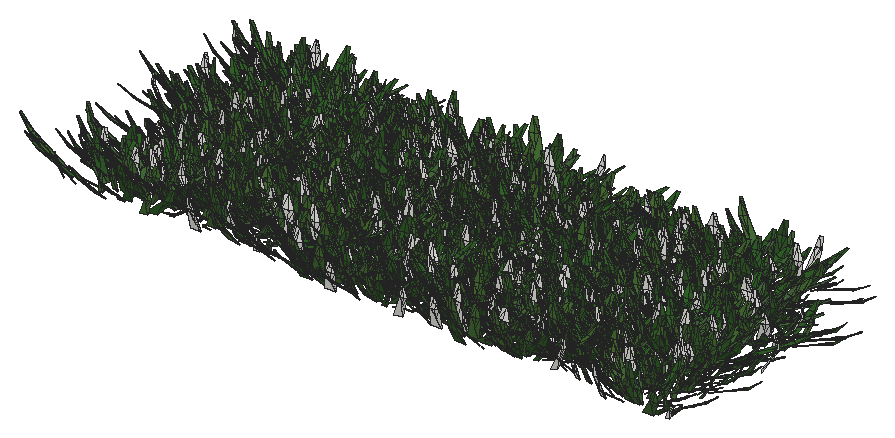
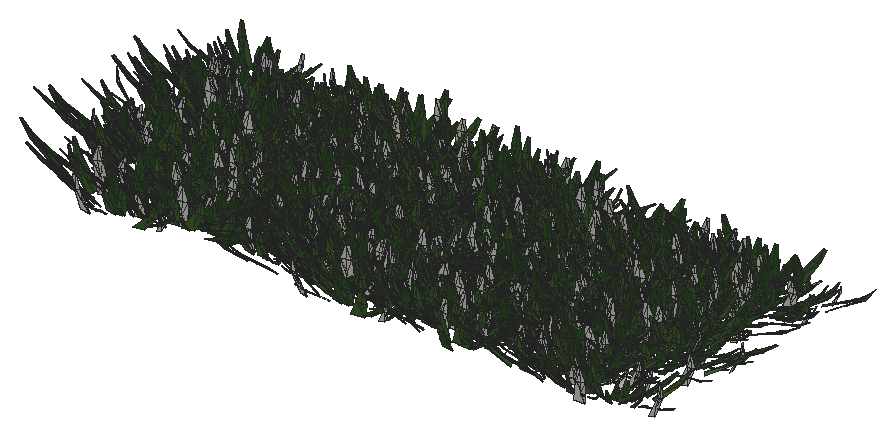
# SketchUp Ruby script. Lengths in inches.
U = 1.inch
M = Sketchup.active_model
def pt(a) = Geom::Point3d.new(a.map { |v| v * U })
def face(e, loops, mat)
  f = e.add_face(loops[0].map { |a| pt(a) })
  loops[1..].each { |l| e.add_face(l.map { |a| pt(a) }).erase! }
  f.material = f.back_material = mat if mat
  f
end
# faces: each face lists its corners as indices into pts; further lists are holes
def faces(e, pts, list, mat = nil) = list.each { |f| face(e, (f[0].is_a?(Array) ? f : [f]).map { |l| l.map { |i| pts[i] } }, mat) }
# xy, xz, yz: faces in a plane at the given z, y or x. An outline is a flat list of corners, or four numbers for a rectangle; further outlines are holes
def ring(l) = l.size == 4 ? [[l[0], l[1]], [l[2], l[1]], [l[2], l[3]], [l[0], l[3]]] : l.each_slice(2).to_a
def flat(e, list, mat, &to3) = list.each { |f| face(e, (f[0].is_a?(Array) ? f : [f]).map { |l| ring(l).map { |u, v| to3.(u, v) } }, mat) }
def xy(e, z, list, mat = nil) = flat(e, list, mat) { |x, y| [x, y, z] }
def xz(e, y, list, mat = nil) = flat(e, list, mat) { |x, z| [x, y, z] }
def yz(e, x, list, mat = nil) = flat(e, list, mat) { |y, z| [x, y, z] }
def lines(e, pts, list) = list.each { |a, b| e.add_line(pt(pts[a]), pt(pts[b])) }
# prism: a flat outline (further loops are holes) pulled along v
def prism(e, loops, v, mat = nil)
  f = face(e, loops, mat); d = Geom::Vector3d.new(v.map { |x| x * U })
  f.pushpull(f.normal.samedirection?(d) ? d.length : -d.length)
end
def box(e, o, s, mat = nil) = prism(e, [[o, [o[0] + s[0], o[1], o[2]], [o[0] + s[0], o[1] + s[1], o[2]], [o[0], o[1] + s[1], o[2]]]], [0, 0, s[2]], mat)
def at(x, y, z, deg = 0) = Geom::Transformation.translation(pt([x, y, z])) * Geom::Transformation.rotation(ORIGIN, Z_AXIS, deg.degrees)
def axes(o, x, y, z) = Geom::Transformation.new([*x, 0, *y, 0, *z, 0, *pt(o).to_a, 1])
def part(name) = M.definitions.add(name)
# library, detail: a bought-in or finely detailed component or shape, given as its bounding box
def library(name, o, s) = part(name).tap { |d| box(d.entities, o, s) }
def detail(e, o, s) = box(e.add_group.entities, o, s)
def put(e, d, t, mat = nil) = e.add_instance(d, t).tap { |i| i.material = mat if mat }
def group(e, t, mat = nil) = e.add_group.tap { |g| g.transformation = t; g.material = mat if mat }.entities
root = M.entities
M.materials.add("Material82").color = [68, 110, 58]
M.materials.add("Material83").color = [48, 90, 38]
M.materials.add("Material84").color = [68, 110, 48]
M.materials.add("Material85").color = [48, 90, 48]
M.materials.add("Material86").color = [58, 110, 58]
M.materials.add("Material87").color = [58, 90, 38]
M.materials.add("Material88").color = [68, 100, 58]
M.materials.add("Material89").color = [48, 100, 38]
c1 = part("grass00")
p = [[-0.6875,0.15,0],[-0.56,0.08,5.52],[-0.04,0.03,2.76],[0.48,-0.02,0],[0.35,-0.02,5.52],[-0.1,-0.14,5.52],
  [-0.12,0.65,8.37],[-0.42,0.65,8.37]]
faces(c1.entities,p,[[0,1,2,3],[3,2,4],[1,5,2],[5,4,2],[1,6,5],[4,5,6],[7,6,1]])
c2 = part("Group16\#1")
put(c2.entities,c1,axes([1.44,-0.61,-0.01],[0.05352,0.12609,0],[-0.10704,0.04543,0.07239],[0.06664,-0.02828,0.11628]),"Material85")
put(c2.entities,c1,axes([0.76,-0.15,-0.01],[0.04676,0.24062,0],[-0.23162,0.04501,0.06642],[0.0652,-0.01267,0.23595]),"Material82")
put(c2.entities,c1,axes([0.79,0.01,-0.01],[-0.00606,0.34651,0],[-0.34381,-0.00602,0.0432],[0.04319,0.00076,0.34386]))
put(c2.entities,c1,axes([1,0.23,-0.01],[-0.07192,0.31144,0],[-0.28722,-0.06632,0.1236],[0.12043,0.02781,0.29478]),"Material84")
put(c2.entities,c1,axes([1.66,0.77,-0.01],[-0.13828,0.29651,0],[-0.21551,-0.1005,0.22471],[0.20365,0.09498,0.23779]),"Material89")
put(c2.entities,c1,axes([0.6875,0.52,-0.01],[-0.18126,0.24051,0],[-0.22746,-0.17142,0.09788],[0.07817,0.05891,0.28481]),"Material84")
put(c2.entities,c1,axes([0.68,0.78,-0.01],[-0.215,0.18688,0],[-0.12385,-0.14248,0.21334],[0.13995,0.16101,0.18878]),"Material82")
put(c2.entities,c1,axes([0.56,1,-0.01],[-0.13756,0.07624,0],[-0.06159,-0.11112,0.0927],[0.04494,0.08108,0.12705]),"Material84")
put(c2.entities,c1,axes([0.2,0.64,-0.01],[-0.23729,0.07254,0],[-0.05711,-0.18681,0.153],[0.04473,0.14632,0.19535]),"Material89")
put(c2.entities,c1,axes([0.0625,0.72,-0.01],[-0.28874,0.02525,0],[-0.02179,-0.24916,0.14647],[0.01276,0.14591,0.25012]),"Material82")
put(c2.entities,c1,axes([-0.08,0.62,-0.01],[-0.34089,-0.04187,0],[0.03255,-0.26504,0.216],[-0.02633,0.21439,0.26703]),"Material89")
put(c2.entities,c1,axes([-0.34,0.98,-0.01],[-0.14314,-0.0493,0],[0.04397,-0.12769,0.06843],[-0.02228,0.0647,0.13505]),"Material89")
put(c2.entities,c1,axes([-0.87,1.45,-0.01],[-0.23488,-0.14114,0],[0.13761,-0.22901,0.06087],[-0.03135,0.05217,0.26717]))
put(c2.entities,c1,axes([-0.72,0.77,-0.01],[-0.14208,-0.13251,0],[0.07209,-0.0773,0.16301],[-0.11118,0.11922,0.1057]),"Material89")
put(c2.entities,c1,axes([-0.62,0.43,-0.01],[-0.14845,-0.21203,0],[0.18654,-0.13061,0.12304],[-0.10079,0.07057,0.22772]),"Material82")
put(c2.entities,c1,axes([-0.68,0.29,-0.01],[-0.13639,-0.32136,0],[0.31723,-0.13464,0.05579],[-0.05136,0.0218,0.34462]),"Material83")
put(c2.entities,c1,axes([-0.64,0.125,-0.01],[-0.0458,-0.23569,0],[0.22124,-0.043,0.08276],[-0.08124,0.01579,0.22538]),"Material86")
put(c2.entities,c1,axes([-1.6,-0.03,-0.01],[0.00576,-0.32897,0],[0.27526,0.00482,0.18018],[-0.18015,-0.00315,0.2753]),"Material84")
put(c2.entities,c1,axes([-1.36,-0.31,-0.01],[0.05718,-0.24765,0],[0.18172,0.04196,0.17267],[-0.16825,-0.03885,0.1865]),"Material89")
put(c2.entities,c1,axes([-1.54,-0.72,-0.01],[0.06537,-0.14017,0],[0.13555,0.06321,0.03939],[-0.0357,-0.01665,0.14956]))
put(c2.entities,c1,axes([-1.19,-0.9,-0.01],[0.09597,-0.12735,0],[0.11214,0.08451,0.07557],[-0.06035,-0.04548,0.14042]),"Material88")
put(c2.entities,c1,axes([-0.47,-0.54,-0.01],[0.11588,-0.10072,0],[0.0618,0.0711,0.12124],[-0.07953,-0.0915,0.0942]))
put(c2.entities,c1,axes([-0.47,-0.84,-0.01],[0.11927,-0.0661,0],[0.06603,0.11913,0.00646],[-0.00313,-0.00565,0.13621]),"Material84")
put(c2.entities,c1,axes([-0.38,-1.24,-0.01],[0.28037,-0.08571,0],[0.0618,0.20215,0.20315],[-0.05939,-0.19428,0.21139]),"Material88")
put(c2.entities,c1,axes([-0.06,-0.66,-0.01],[0.22719,-0.01987,0],[0.01247,0.14255,0.17758],[-0.01547,-0.17691,0.1431]),"Material87")
put(c2.entities,c1,axes([0.11,-0.89,-0.01],[0.14882,0.01828,0],[-0.01058,0.08611,0.12229],[0.01491,-0.12138,0.08676]),"Material85")
put(c2.entities,c1,axes([0.25,-0.72,-0.01],[0.20481,0.07053,0],[-0.06206,0.18022,0.10291],[0.03351,-0.0973,0.1906]),"Material85")
put(c2.entities,c1,axes([0.85,-1.42,-0.01],[0.16481,0.09904,0],[-0.09472,0.15762,0.05616],[0.02893,-0.04814,0.18389]),"Material84")
put(c2.entities,c1,axes([1.01,-1.09,-0.01],[0.21858,0.20385,0],[-0.17495,0.1876,0.15339],[0.10462,-0.11218,0.25652]),"Material89")
put(c2.entities,c1,axes([1.01,-0.71,-0.01],[0.08733,0.12473,0],[-0.06445,0.04512,0.13037],[0.1068,-0.07477,0.07867]),"Material85")
c3 = part("Group15\#1")
put(c3.entities,c2,at(0,0,0))
c4 = part("3darcstudiotree_grass00\#1")
put(c4.entities,c3,at(0,0,0))
put(root,c4,axes([773.21,342.86,-34.17],[3.14963,-1.20842,0],[2.29792,0.93151,-0.01443],[0.07601,0.03081,1.86565]))
put(root,c4,axes([774.36,356.8,-34.17],[-4.00454,-0.52801,0],[1.05814,-1.24816,-0.00172],[0.00311,-0.00367,1.42531]))
put(root,c4,axes([774.46,343.67,-34.17],[-1.0046,-1.54951,0],[3.94346,-0.39764,-0.04783],[0.24428,-0.02463,1.6084]))
put(root,c4,axes([772.96,366.74,-34.17],[2.75664,0.78459,0],[-2.60411,1.42301,-0.01696],[-0.0547,0.02989,1.8379]))
put(root,c4,axes([773.18,355.92,-34.17],[1.57656,1.15501,0],[-3.7913,0.80487,-0.00648],[-0.02974,0.00631,1.68262]))
put(root,c4,axes([775.48,345.66,-34.17],[-0.37683,-1.42813,0],[4.6236,-0.18974,-0.00351],[0.01488,-0.00061,1.48465]))
put(root,c4,axes([773.68,340.73,-34.17],[4.54007,0.12562,0],[-0.30482,1.71344,-0.05051],[-0.02069,0.11631,1.91076]))
put(root,c4,axes([775.09,350.05,-34.17],[1.62707,-1.18617,0],[3.8873,0.82932,-0.03985],[0.15889,0.0339,1.5017]))
put(root,c4,axes([774.64,359.32,-34.17],[4.17569,0.70475,0],[-1.86329,1.71705,-0.06274],[-0.13365,0.12316,1.92197]))
put(root,c4,axes([777.05,351.61,-34.17],[-3.80347,-0.79702,0],[1.88494,-1.39901,-0.03648],[0.10192,-0.07565,1.79293]))
put(root,c4,axes([776.98,349.31,-34.17],[-2.17021,-1.46243,0],[2.84473,-0.65657,-0.0221],[0.14072,-0.03248,1.82262]))
put(root,c4,axes([778.55,353.74,-34.17],[-2.18591,-1.17845,0],[3.11783,-0.89946,-0.02018],[0.10185,-0.02938,1.81061]))
put(root,c4,axes([777.24,367.79,-34.17],[4.09864,-0.14348,0],[0.37168,1.65134,-0.01913],[0.00999,0.04439,1.86132]))
put(root,c4,axes([777.85,355.56,-34.17],[-1.78032,1.61918,0],[-3.86174,-0.66038,-0.00354],[-0.01693,-0.0029,1.64409]))
put(root,c4,axes([778.8,342.72,-34.17],[3.03313,0.50579,0],[-1.37798,1.28522,-0.04149],[-0.11611,0.10829,1.90578]))
put(root,c4,axes([778.73,343.85,-34.17],[4.0409,0.57443,0],[-1.45336,1.59011,-0.05978],[-0.09434,0.10321,1.49495]))
put(root,c4,axes([778.6,364.67,-34.17],[3.09052,1.16305,0],[-2.75216,1.13741,-0.00767],[-0.03246,0.01341,1.8325]))
put(root,c4,axes([779.77,346.72,-34.17],[1.55138,-1.30688,0],[2.99369,0.55272,-0.04141],[0.29892,0.05519,1.97468]))
put(root,c4,axes([779.62,360.0625,-34.17],[4.14328,-0.46419,0],[1.00154,1.39037,-0.02465],[0.03463,0.04808,1.41248]))
put(root,c4,axes([780.14,358.2,-34.17],[-0.77153,1.33479,0],[-3.28421,-0.29525,-0.03421],[-0.24787,-0.02228,1.87625]))
put(root,c4,axes([780.48,361.74,-34.17],[-1.91367,1.54924,0],[-4.25661,-0.81775,-0.00711],[-0.02422,-0.00465,1.34501]))
put(root,c4,axes([781.09,366.36,-34.17],[3.43874,0.27286,0],[-0.6732,1.31953,-0.0192],[-0.02432,0.04768,1.64321]))
put(root,c4,axes([782.6,343.8125,-34.17],[-4.1133,-0.05921,0],[0.15009,-1.6218,-0.04384],[0.00865,-0.09349,1.66887]))
put(root,c4,axes([783.42,341.69,-34.17],[-3.5543,0.89209,0],[-1.79933,-1.11498,-0.04609],[-0.16829,-0.10428,1.7083]))
put(root,c4,axes([784.125,346.45,-34.17],[-2.34222,-1.01748,0],[3.28821,-1.17726,-0.05879],[0.21723,-0.07777,1.66118]))
put(root,c4,axes([783.17,363.76,-34.17],[3.65348,-0.50094,0],[1.24961,1.41744,-0.02118],[0.04225,0.04793,1.73224]))
put(root,c4,axes([784.34,359.43,-34.17],[-0.28709,-1.61704,0],[4.14071,-0.11434,-0.04142],[0.22933,-0.00633,1.72685]))
put(root,c4,axes([783.02,366.19,-34.17],[1.27855,1.29921,0],[-4.02019,0.61532,-0.04732],[-0.19364,0.02964,1.41896]))
put(root,c4,axes([783.54,350.0625,-34.17],[-1.96915,1.54328,0],[-4.06414,-0.80652,-0.00338],[-0.01619,-0.00321,1.82725]))
put(root,c4,axes([785.07,349.04,-34.17],[-3.56597,0.54096,0],[-1.21057,-1.24113,-0.01112],[-0.02689,-0.02757,1.70172]))
put(root,c4,axes([783.88,361.6,-34.17],[3.55843,0.77732,0],[-2.07504,1.47739,-0.02111],[-0.0608,0.04329,1.90804]))
put(root,c4,axes([784.41,357.15,-34.17],[4.24476,0.21314,0],[-0.43337,1.34235,-0.04636],[-0.04216,0.1306,1.85211]))
put(root,c4,axes([786.4,354.75,-34.17],[-3.8899,-0.78174,0],[2.11548,-1.63718,-0.02171],[0.04442,-0.03438,1.57387]))
put(root,c4,axes([786.41,353.11,-34.17],[3.28347,0.12106,0],[-0.38901,1.64106,-0.04931],[-0.02254,0.09507,1.538]))
put(root,c4,axes([789.21,354.72,-34.17],[-3.55041,0.9087,0],[-2.02381,-1.22981,-0.02727],[-0.0752,-0.0457,1.41127]))
put(root,c4,axes([788.76,359.69,-34.17],[1.12356,1.5327,0],[-3.46853,0.39546,-0.04889],[-0.25471,0.02904,1.46761]))
put(root,c4,axes([790.3125,344.57,-34.17],[1.64327,-1.14246,0],[4.09949,0.91708,-0.03953],[0.17253,0.0386,1.77239]))
put(root,c4,axes([789.09,342.6,-34.17],[0.41174,1.83159,0],[-3.96576,0.13865,-0.0152],[-0.08151,0.00285,1.60635]))
put(root,c4,axes([791.24,348.04,-34.17],[0.23576,-1.73441,0],[4.70751,0.09952,-0.00697],[0.03732,0.00079,1.89407]))
put(root,c4,axes([791.03,352.72,-34.17],[-3.49986,-0.57002,0],[1.44663,-1.38143,-0.04671],[0.11633,-0.11108,1.85324]))
put(root,c4,axes([790.11,346.12,-34.17],[0.9145,1.75116,0],[-3.69114,0.2998,-0.03105],[-0.20233,0.01643,1.87912]))
put(root,c4,axes([790.38,350.85,-34.17],[1.28043,1.73979,0],[-3.30316,0.37809,-0.03743],[-0.19576,0.02241,1.40382]))
put(root,c4,axes([790.87,361.54,-34.17],[2.41483,0.92576,0],[-3.06998,1.24547,-0.04673],[-0.14351,0.05822,1.45453]))
put(root,c4,axes([791.32,363.54,-34.17],[4.28624,-0.48224,0],[1.29741,1.79351,-0.04256],[0.05122,0.07081,1.55488]))
put(root,c4,axes([791.65,365.39,-34.17],[0.63995,1.63517,0],[-3.50377,0.21327,-0.04631],[-0.28502,0.01735,1.65491]))
put(root,c4,axes([792.12,357.61,-34.17],[4.08655,-0.74198,0],[1.4526,1.2443,-0.00355],[0.00912,0.00781,1.60125]))
put(root,c4,axes([792.1,367.56,-34.17],[1.05791,1.29898,0],[-3.4169,0.4328,-0.04361],[-0.24845,0.03147,1.60948]))
put(root,c4,axes([793.73,355.39,-34.17],[-0.24051,-1.38856,0],[3.98568,-0.10737,-0.04502],[0.19517,-0.00526,1.30109]))
put(root,c4,axes([794.77,344.86,-34.17],[1.00632,-1.60929,0],[3.83281,0.37276,-0.00763],[0.0458,0.00445,1.82848]))
put(root,c4,axes([795.37,350.2,-34.17],[-2.49579,-0.85332,0],[2.16334,-0.98408,-0.00893],[0.04692,-0.02134,1.98619]))
put(root,c4,axes([795.32,364.02,-34.17],[2.15184,-1.02148,0],[3.44742,1.1295,-0.00974],[0.03611,0.01183,1.619]))
put(root,c4,axes([795.6875,352.47,-34.17],[-3.56783,-0.13568,0],[0.42403,-1.73414,-0.0118],[0.00459,-0.01877,1.34216]))
put(root,c4,axes([795.03,357,-34.17],[4.22834,-0.67564,0],[1.61938,1.57623,-0.01357],[0.03127,0.03043,1.98263]))
put(root,c4,axes([795.31,346.92,-34.17],[3.42011,0.99957,0],[-2.24279,1.19352,-0.03152],[-0.09807,0.05219,1.47514]))
put(root,c4,axes([797.41,341.58,-34.17],[-0.92987,-1.7368,0],[3.78348,-0.31505,-0.00703],[0.03581,-0.00298,1.50812]))
put(root,c4,axes([796.01,358.77,-34.17],[3.74003,-0.3626,0],[0.86697,1.39078,-0.02888],[0.04393,0.07047,1.73467]))
put(root,c4,axes([797.61,349.15,-34.17],[-2.16285,-1.07783,0],[3.1191,-0.97346,-0.00813],[0.02825,-0.00882,1.32168]))
put(root,c4,axes([796.02,366.05,-34.17],[2.54513,1.12368,0],[-2.54126,0.89522,-0.01423],[-0.07597,0.02676,1.82816]))
put(root,c4,axes([797.03,362.52,-34.17],[-2.35271,1.42324,0],[-3.1761,-0.81658,-0.00573],[-0.02769,-0.00712,1.63969]))
put(root,c4,axes([799.12,362.21,-34.17],[-2.99545,-1.01525,0],[2.44315,-1.12112,-0.00129],[0.00439,-0.00201,1.46122]))
put(root,c4,axes([799.49,340.5,-34.17],[-4.11359,0.33172,0],[-0.73599,-1.4195,-0.0347],[-0.04072,-0.07853,1.61275]))
put(root,c4,axes([800.74,355.09,-34.17],[-1.26006,-1.32624,0],[4.43512,-0.65537,-0.00645],[0.02239,-0.00331,1.31612]))
put(root,c4,axes([799.14,347.21,-34.17],[0.26665,1.72733,0],[-3.78087,0.09078,-0.02381],[-0.14887,0.00357,1.77807]))
put(root,c4,axes([800.39,356.875,-34.17],[0.22416,-1.4452,0],[4.13727,0.09981,-0.05271],[0.23324,0.00563,1.37729]))
put(root,c4,axes([800.16,341.31,-34.17],[2.00643,-1.16557,0],[2.7626,0.73963,-0.03969],[0.18592,0.04978,1.41714]))
put(root,c4,axes([801.0625,353.65,-34.17],[-2.85144,-1.16634,0],[2.50888,-0.95396,-0.03577],[0.14723,-0.05598,1.49339]))
put(root,c4,axes([799.83,350.85,-34.17],[1.02208,1.31259,0],[-4.10151,0.49672,-0.03259],[-0.17155,0.02078,1.77089]))
put(root,c4,axes([799.83,364.71,-34.17],[2.93363,1.22701,0],[-2.56818,0.95498,-0.02839],[-0.14721,0.05474,1.88589]))
put(root,c4,axes([801.75,360.3,-34.17],[-0.17296,-1.31916,0],[4.52056,-0.09218,-0.00424],[0.01978,-0.0004,1.58408]))
put(root,c4,axes([802.88,348.625,-34.17],[-4.36692,-0.69342,0],[1.6396,-1.60594,-0.01703],[0.03175,-0.0311,1.64249]))
put(root,c4,axes([802.89,365.94,-34.17],[-4.04807,0.23611,0],[-0.60438,-1.61163,-0.04443],[-0.03837,-0.10233,1.82802]))
put(root,c4,axes([801.43,344.16,-34.17],[3.28108,0.9921,0],[-2.06723,1.06332,-0.03117],[-0.09708,0.04994,1.30357]))
put(root,c4,axes([804.91,360.25,-34.17],[-3.17197,-0.90891,0],[2.49685,-1.35522,-0.03763],[0.13517,-0.07337,1.94544]))
put(root,c4,axes([805.24,351.03,-34.17],[-3.35579,-1.19548,0],[2.90415,-1.2679,-0.0585],[0.2305,-0.10063,1.90866]))
put(root,c4,axes([805.1,368.26,-34.17],[1.68348,-1.42,0],[3.90393,0.71983,-0.01397],[0.0682,0.01258,1.74087]))
put(root,c4,axes([804.65,358.17,-34.17],[-1.26035,1.30994,0],[-3.37363,-0.50484,-0.03389],[-0.19382,-0.029,1.65454]))
put(root,c4,axes([805.84,340.4,-34.17],[-3.39608,-0.38473,0],[1.21289,-1.66516,-0.05258],[0.08123,-0.11153,1.84274]))
put(root,c4,axes([806.27,347.85,-34.17],[-0.07574,-1.47303,0],[4.38332,-0.03505,-0.05384],[0.21677,-0.00173,1.32332]))
put(root,c4,axes([806.24,352.84,-34.17],[-3.58969,-0.07657,0],[0.18796,-1.37056,-0.00522],[0.00152,-0.01105,1.40302]))
put(root,c4,axes([806.32,364.52,-34.17],[-3.78052,0.58265,0],[-1.19847,-1.20943,-0.02866],[-0.07958,-0.08031,1.88291]))
put(root,c4,axes([807.08,355.84,-34.17],[-3.3619,-0.88005,0],[2.60897,-1.55009,-0.03911],[0.08798,-0.05227,1.43856]))
put(root,c4,axes([806.53,345.96,-34.17],[-0.00326,-1.3732,0],[3.39922,-0.00125,-0.0371],[0.2688,-0.0001,1.84609]))
put(root,c4,axes([807.31,365.9,-34.17],[-2.81078,-0.75848,0],[2.18011,-1.25652,-0.01797],[0.04803,-0.02768,1.36964]))
put(root,c4,axes([806.39,344.97,-34.17],[3.61578,-1.02121,0],[2.66994,1.47029,-0.04389],[0.14306,0.07878,1.92393]))
put(root,c4,axes([807.4375,342.71,-34.17],[3.76801,-0.42175,0],[1.14915,1.59678,-0.03157],[0.04846,0.06733,1.77323]))
put(root,c4,axes([807.74,361.52,-34.17],[2.09185,1.03032,0],[-2.8732,0.90727,-0.01526],[-0.08429,0.02662,1.9517]))
put(root,c4,axes([810.78,351.16,-34.17],[-1.37112,-1.31689,0],[3.73876,-0.60543,-0.04381],[0.2334,-0.0378,1.74465]))
put(root,c4,axes([811.4,364.17,-34.17],[-0.8424,-1.2576,0],[4.34376,-0.45254,-0.01354],[0.07406,-0.00772,1.90468]))
put(root,c4,axes([810.58,358.94,-34.17],[3.65327,1.04493,0],[-2.10749,1.14596,-0.01189],[-0.03901,0.02121,1.50367]))
put(root,c4,axes([811.83,354.6,-34.17],[-2.51613,1.14478,0],[-2.79457,-0.95529,-0.04719],[-0.16752,-0.05727,1.30223]))
put(root,c4,axes([810.875,365.96,-34.17],[3.43468,1.02641,0],[-2.59272,1.34938,-0.0181],[-0.04577,0.02382,1.34745]))
put(root,c4,axes([812.64,341.85,-34.17],[-4.19905,0.34301,0],[-0.96105,-1.82979,-0.05761],[-0.05651,-0.10759,1.71741]))
put(root,c4,axes([811.83,362.37,-34.17],[3.21656,-1.06764,0],[2.25071,1.05463,-0.04982],[0.17505,0.08203,1.4295]))
put(root,c4,axes([813.27,345.05,-34.17],[0.12061,-1.58998,0],[4.18389,0.04936,-0.01737],[0.08566,0.00101,1.54781]))
put(root,c4,axes([813.84,356.91,-34.17],[-3.70247,-0.49757,0],[1.50858,-1.74588,-0.06303],[0.09341,-0.1081,1.61067]))
put(root,c4,axes([812.83,347.21,-34.17],[-0.34365,1.56469,0],[-3.45908,-0.11816,-0.04948],[-0.26965,-0.00921,1.42361]))
put(root,c4,axes([812.38,352.77,-34.17],[1.76415,1.1719,0],[-3.51067,0.82196,-0.05173],[-0.20066,0.04698,1.38038]))
put(root,c4,axes([813.14,348.74,-34.17],[4.55756,-0.02191,0],[0.04205,1.36049,-0.04731],[0.00354,0.1146,1.58849]))
put(root,c4,axes([817.28,363.75,-34.17],[-3.74528,-0.54225,0],[1.29092,-1.38673,-0.02574],[0.04375,-0.047,1.38465]))
put(root,c4,axes([817.17,360.06,-34.17],[-3.91187,0.00169,0],[-0.00401,-1.44027,-0.04481],[-0.00031,-0.10997,1.70362]))
put(root,c4,axes([818.36,348.83,-34.17],[-3.9934,-0.49353,0],[1.06998,-1.34652,-0.00157],[0.00241,-0.00304,1.37913]))
put(root,c4,axes([818.3,340.58,-34.17],[-1.39646,-1.43145,0],[3.7454,-0.56828,-0.0371],[0.22587,-0.03427,1.96201]))
put(root,c4,axes([817.2,365.71,-34.17],[2.25108,1.29367,0],[-3.07657,0.83262,-0.0512],[-0.2098,0.05678,1.38975]))
put(root,c4,axes([817.89,357.38,-34.17],[-1.78787,1.37846,0],[-3.47115,-0.7002,-0.05082],[-0.20934,-0.04223,1.35221]))
put(root,c4,axes([817.17,355.66,-34.17],[3.1901,1.34772,0],[-3.0794,1.13365,-0.04297],[-0.19725,0.07262,1.98261]))
put(root,c4,axes([818.64,361.08,-34.17],[-3.49916,1.06741,0],[-2.60054,-1.32589,-0.05181],[-0.14447,-0.07366,1.45196]))
put(root,c4,axes([818.84,353.76,-34.17],[-3.70101,0.79314,0],[-2.22235,-1.61286,-0.04664],[-0.10432,-0.07571,1.63424]))
put(root,c4,axes([817.55,342.17,-34.17],[1.4538,1.50227,0],[-4.10712,0.61817,-0.00597],[-0.03083,0.00464,1.82255]))
put(root,c4,axes([818.8125,346.49,-34.17],[-1.85188,1.07885,0],[-3.29338,-0.87924,-0.00267],[-0.01201,-0.00321,1.62102]))
put(root,c4,axes([819.55,350.35,-34.17],[2.80724,-1.17226,0],[3.04027,1.13235,-0.05261],[0.16943,0.06311,1.38839]))
put(root,c4,axes([818.88,344.08,-34.17],[3.28196,0.81984,0],[-2.45781,1.53025,-0.01012],[-0.02495,0.01554,1.58691]))
put(root,c4,axes([821.52,348.75,-34.17],[-0.83235,-1.28841,0],[3.31595,-0.33318,-0.03395],[0.19708,-0.0198,1.53644]))
put(root,c4,axes([821.86,352.37,-34.17],[-0.43709,-1.41781,0],[4.63894,-0.22243,-0.04217],[0.16902,-0.0081,1.41426]))
put(root,c4,axes([821.29,357.96,-34.17],[3.88367,-0.39615,0],[1.13822,1.73547,-0.04841],[0.06323,0.0964,1.77682]))
put(root,c4,axes([822.74,342.02,-34.17],[-0.85576,-1.5606,0],[4.52661,-0.38605,-0.05631],[0.21879,-0.01866,1.37991]))
put(root,c4,axes([822.99,355.05,-34.17],[-2.86852,-0.72551,0],[1.94813,-1.19796,-0.01822],[0.05809,-0.03572,1.59761]))
put(root,c4,axes([822.76,345.8,-34.17],[-3.59941,0.74413,0],[-1.52837,-1.14979,-0.02232],[-0.06679,-0.05025,1.59039]))
put(root,c4,axes([821.39,359.95,-34.17],[1.48622,1.27925,0],[-3.96463,0.71638,-0.00338],[-0.01448,0.00262,1.53978]))
put(root,c4,axes([823.375,363.74,-34.17],[1.63817,-1.67164,0],[3.7967,0.57868,-0.011],[0.05001,0.00762,1.48653]))
put(root,c4,axes([823.81,340.65,-34.17],[-2.82588,-0.78458,0],[2.18733,-1.22531,-0.03828],[0.15336,-0.08591,1.98208]))
put(root,c4,axes([824.82,345.03,-34.17],[-1.60743,-1.14355,0],[3.95374,-0.86436,-0.00731],[0.03731,-0.00816,1.97847]))
put(root,c4,axes([824.85,361.95,-34.17],[-3.32772,0.28661,0],[-0.75668,-1.36642,-0.01018],[-0.01111,-0.02006,1.35975]))
put(root,c4,axes([823.875,350.23,-34.17],[3.98724,0.20884,0],[-0.61603,1.82924,-0.05242],[-0.03685,0.10943,1.87281]))
put(root,c4,axes([824.875,365.46,-34.17],[-0.30333,1.33059,0],[-3.40704,-0.1208,-0.0349],[-0.19211,-0.00681,1.41691]))
put(root,c4,axes([828.125,342.5625,-34.17],[-2.807,-0.90771,0],[2.30635,-1.10925,-0.04795],[0.15506,-0.07458,1.39039]))
put(root,c4,axes([827.18,345.74,-34.17],[3.2807,-0.61041,0],[1.81668,1.51857,-0.02435],[0.05518,0.04613,1.69455]))
put(root,c4,axes([828.37,360.95,-34.17],[-1.43959,-1.62411,0],[3.7168,-0.5124,-0.03865],[0.23963,-0.03303,1.9383]))
put(root,c4,axes([829.0625,363.94,-34.17],[-3.81782,0.15844,0],[-0.49654,-1.86087,-0.00853],[-0.00435,-0.0163,1.7318]))
put(root,c4,axes([829.76,349.4,-34.17],[-3.12571,-0.7496,0],[2.43282,-1.57777,-0.06276],[0.13907,-0.09019,1.49667]))
put(root,c4,axes([828.14,344.7,-34.17],[2.97603,0.7742,0],[-2.07464,1.24033,-0.03997],[-0.14341,0.08574,1.84008]))
put(root,c4,axes([829.98,352.43,-34.17],[-2.31531,-0.95478,0],[2.79879,-1.05558,-0.03327],[0.10847,-0.04091,1.30962]))
put(root,c4,axes([830.06,357.14,-34.17],[-3.94904,-0.28889,0],[0.74698,-1.58808,-0.00704],[0.00779,-0.01657,1.86241]))
put(root,c4,axes([828.96,366.4375,-34.17],[-1.72673,1.11938,0],[-3.66172,-0.8785,-0.02284],[-0.09991,-0.02397,1.64481]))
put(root,c4,axes([829.37,350.12,-34.17],[-0.65898,1.54379,0],[-3.85922,-0.25621,-0.04712],[-0.21087,-0.014,1.33133]))
put(root,c4,axes([828.97,355.43,-34.17],[1.80555,1.12349,0],[-3.92794,0.98179,-0.01772],[-0.05919,0.0148,1.37883]))
put(root,c4,axes([830.79,358.93,-34.17],[-2.45667,1.24552,0],[-3.48685,-1.06965,-0.01031],[-0.04097,-0.01257,1.66779]))
put(root,c4,axes([832.32,350.98,-34.17],[-1.11481,1.68554,0],[-3.85911,-0.39697,-0.04083],[-0.25467,-0.0262,1.92702]))
put(root,c4,axes([832.84,365.85,-34.17],[3.83562,-0.64652,0],[1.50566,1.38929,-0.01454],[0.02594,0.02394,1.30369]))
put(root,c4,axes([833.68,363.77,-34.17],[-3.30618,0.81403,0],[-2.41899,-1.52802,-0.02972],[-0.07466,-0.04716,1.62371]))
put(root,c4,axes([835.24,346.76,-34.17],[-3.64839,-0.0594,0],[0.18827,-1.79867,-0.05407],[0.01098,-0.10487,1.68402]))
put(root,c4,axes([833.8,341.67,-34.17],[2.37064,0.94684,0],[-3.28047,1.27743,-0.04002],[-0.15051,0.05861,1.82631]))
put(root,c4,axes([834.76,361.67,-34.17],[-3.05865,1.0781,0],[-2.78611,-1.22937,-0.02716],[-0.07662,-0.03381,1.32671]))
put(root,c4,axes([835.88,359.27,-34.17],[-2.13062,-1.66467,0],[3.82642,-0.7617,-0.02075],[0.09652,-0.01921,1.67433]))
put(root,c4,axes([835.83,348.76,-34.17],[-4.39804,-0.22301,0],[0.45888,-1.40747,-0.03967],[0.03344,-0.10258,1.78282]))
put(root,c4,axes([835.19,368.15,-34.17],[2.97779,-1.31333,0],[2.93322,1.03437,-0.03435],[0.15944,0.05623,1.83666]))
put(root,c4,axes([836.13,355.65,-34.17],[-3.86294,0.12208,0],[-0.37038,-1.82279,-0.02116],[-0.00872,-0.04291,1.79229]))
put(root,c4,axes([836.2,357.86,-34.17],[4.62049,-0.36242,0],[0.91883,1.82189,-0.02703],[0.02558,0.05072,1.71263]))
put(root,c4,axes([836.09,352.21,-34.17],[4.4065,0.29877,0],[-0.73465,1.68517,-0.00744],[-0.00712,0.01634,1.83611]))
put(root,c4,axes([836.17,344.4,-34.17],[2.92133,1.34194,0],[-2.9494,0.99861,-0.03135],[-0.14252,0.04825,1.74596]))
put(root,c4,axes([837.94,359.25,-34.17],[-4.37191,-0.09188,0],[0.22077,-1.63377,-0.04256],[0.01218,-0.09013,1.67228]))
put(root,c4,axes([838.57,351,-34.17],[-0.6545,-1.64207,0],[4.59681,-0.28496,-0.0381],[0.20859,-0.01293,1.93318]))
put(root,c4,axes([837.96,345.98,-34.17],[3.15887,-0.80876,0],[1.92191,1.16751,-0.02789],[0.09845,0.05981,1.71527]))
put(root,c4,axes([838.79,347.97,-34.17],[-3.60106,0.31713,0],[-0.9107,-1.60836,-0.00123],[-0.0017,-0.003,1.99006]))
put(root,c4,axes([838.66,344.0625,-34.17],[1.90217,1.207,0],[-3.00756,0.73717,-0.00184],[-0.00944,0.00231,1.60144]))
put(root,c4,axes([839.58,340.08,-34.17],[-1.8058,1.22943,0],[-3.0103,-0.68768,-0.02138],[-0.11593,-0.02648,1.63406]))
put(root,c4,axes([839.57,357.88,-34.17],[-1.11998,1.52641,0],[-4.36702,-0.49835,-0.06381],[-0.30025,-0.03426,1.66913]))
